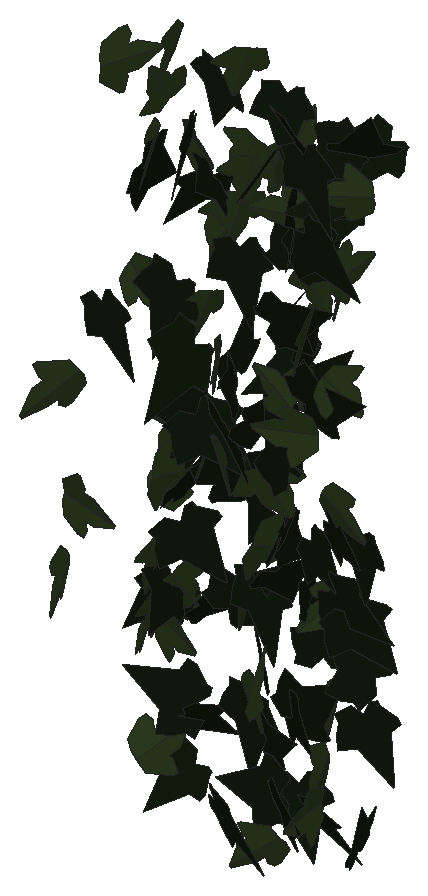
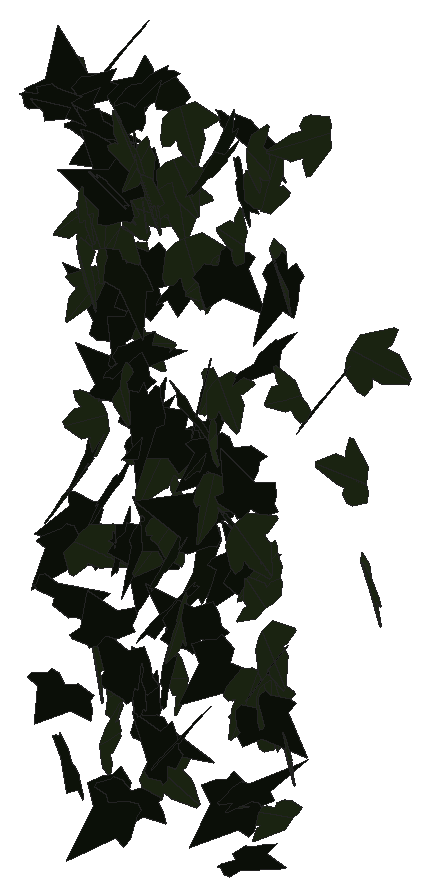
# SketchUp Ruby script. Lengths in inches.
U = 1.inch
M = Sketchup.active_model
def pt(a) = Geom::Point3d.new(a.map { |v| v * U })
def face(e, loops, mat)
  f = e.add_face(loops[0].map { |a| pt(a) })
  loops[1..].each { |l| e.add_face(l.map { |a| pt(a) }).erase! }
  f.material = f.back_material = mat if mat
  f
end
# faces: each face lists its corners as indices into pts; further lists are holes
def faces(e, pts, list, mat = nil) = list.each { |f| face(e, (f[0].is_a?(Array) ? f : [f]).map { |l| l.map { |i| pts[i] } }, mat) }
# xy, xz, yz: faces in a plane at the given z, y or x. An outline is a flat list of corners, or four numbers for a rectangle; further outlines are holes
def ring(l) = l.size == 4 ? [[l[0], l[1]], [l[2], l[1]], [l[2], l[3]], [l[0], l[3]]] : l.each_slice(2).to_a
def flat(e, list, mat, &to3) = list.each { |f| face(e, (f[0].is_a?(Array) ? f : [f]).map { |l| ring(l).map { |u, v| to3.(u, v) } }, mat) }
def xy(e, z, list, mat = nil) = flat(e, list, mat) { |x, y| [x, y, z] }
def xz(e, y, list, mat = nil) = flat(e, list, mat) { |x, z| [x, y, z] }
def yz(e, x, list, mat = nil) = flat(e, list, mat) { |y, z| [x, y, z] }
def lines(e, pts, list) = list.each { |a, b| e.add_line(pt(pts[a]), pt(pts[b])) }
# prism: a flat outline (further loops are holes) pulled along v
def prism(e, loops, v, mat = nil)
  f = face(e, loops, mat); d = Geom::Vector3d.new(v.map { |x| x * U })
  f.pushpull(f.normal.samedirection?(d) ? d.length : -d.length)
end
def box(e, o, s, mat = nil) = prism(e, [[o, [o[0] + s[0], o[1], o[2]], [o[0] + s[0], o[1] + s[1], o[2]], [o[0], o[1] + s[1], o[2]]]], [0, 0, s[2]], mat)
def at(x, y, z, deg = 0) = Geom::Transformation.translation(pt([x, y, z])) * Geom::Transformation.rotation(ORIGIN, Z_AXIS, deg.degrees)
def axes(o, x, y, z) = Geom::Transformation.new([*x, 0, *y, 0, *z, 0, *pt(o).to_a, 1])
def part(name) = M.definitions.add(name)
# library, detail: a bought-in or finely detailed component or shape, given as its bounding box
def library(name, o, s) = part(name).tap { |d| box(d.entities, o, s) }
def detail(e, o, s) = box(e.add_group.entities, o, s)
def put(e, d, t, mat = nil) = e.add_instance(d, t).tap { |i| i.material = mat if mat }
def group(e, t, mat = nil) = e.add_group.tap { |g| g.transformation = t; g.material = mat if mat }.entities
root = M.entities
M.materials.add("efeu1").color = [18, 25, 13]
M.materials.add("efeu2").color = [43, 57, 29]
c1 = part("ivyleaf_9")
p = [[1.54,2.16,1.25],[1.36,2.04,1.19],[-0.21,0.99,0.68],[-0.71,1.11,0.82],[-0.85,0.86,0.67],[-0.8,0.17,0.21],
  [-0.9,-0.01,0.1],[-0.67,-0.16,-0.02],[-0.08,-0.08,-0.05],[-0.03,-0.6,-0.4],[0.65,-0.88,-0.66],[0.83,-0.6,-0.49],
  [1.29,-0.42,-0.43],[1.8125,-0.07,-0.26],[1.21,0.44,0.15]]
faces(c1.entities,p,[[0,1,2,3,4,5,6,7,8,9,10,11,12,13,14]],"efeu1")
c2 = part("ivyleaf_10")
p = [[0,0.5,-0.03],[-0.0625,2.02,-0.43],[-0.19,2.01,-0.46],[-0.54,1.05,-0.29],[-0.52,0.625,-0.18],[-0.83,0.76,-0.28],
  [-1.16,0.64,-0.33],[-1.15,0.33,-0.24],[-0.77,-0.39,0.02],[-0.3,-0.51,0.16],[0.04,-0.48,0.23],[-0.02,2.01,-0.4375],
  [-0.06,2.01,-0.43],[0.04,-0.49,0.23],[0.67,-0.49,0.14],[1.38,0.36,-0.2],[1.375,0.51,-0.24],[0.81,0.65,-0.19],
  [0.62,0.59,-0.15],[0.6,1.09,-0.28],[0.5,1.23,-0.31]]
faces(c2.entities,p,[[0,1,2,3,4,5,6,7,8,9,10],[11,12,0,13,14,15,16,17,18,19,20]],"efeu2")
put(root,c1,axes([575.81,114.26,235.49],[-1.308,-0.18364,-0.30773],[0.30435,0.04552,-1.32082],[0.18917,-1.34294,-0.00269]))
put(root,c1,axes([577.29,114.21,213.41],[1.13881,-0.56952,-0.46488],[-0.40509,0.22917,-1.27308],[0.61349,1.2085,0.02233]))
put(root,c2,axes([577.51,116.32,217.81],[0.87571,-0.89625,-0.03596],[0.02653,-0.02436,1.25304],[-0.89657,-0.87611,0.00195]))
put(root,c2,axes([566.08,117.8,228.98],[-0.23963,-0.68527,1.0215],[-0.33171,-0.96615,-0.72595],[1.1845,-0.4092,0.00335]))
put(root,c2,axes([566.27,117.97,222.96],[0.05434,-0.11388,1.24145],[1.24187,0.11376,-0.04392],[-0.10916,1.23742,0.11829]))
put(root,c2,axes([565.16,118.66,218.99],[0.88338,-0.86872,0.00346],[0.01078,0.00603,-1.23891],[0.86866,0.88336,0.01186]))
put(root,c2,axes([578.02,119.21,229.83],[0.07725,-0.00335,-1.1407],[-1.13047,-0.15301,-0.0761],[-0.15244,1.13303,-0.01366]))
put(root,c2,axes([577.11,121.18,210.1],[-0.02306,0.08063,-1.16362],[-0.17029,-1.15161,-0.07642],[-1.15391,0.16833,0.03453]))
put(root,c1,axes([575.34,121.03,209.32],[0.20393,-0.35155,1.12904],[0.49116,-1.01702,-0.40539],[1.07568,0.53102,-0.02895]))
put(root,c2,axes([572.17,120.58,226.52],[-0.60926,0.6898,-0.52411],[0.35827,-0.38277,-0.92024],[-0.78877,-0.70666,-0.01315]))
put(root,c1,axes([576.48,121.25,242],[0.52528,-1.1541,-0.11164],[-0.03269,0.10778,-1.26793],[1.15902,0.52608,0.01483]))
put(root,c1,axes([574.41,120.85,240.82],[-0.57801,0.89862,-0.10934],[0.06117,-0.09065,-1.06846],[-0.90318,-0.58123,-0.00239]))
put(root,c2,axes([574.33,121.5,207.34],[-0.49806,-0.4723,0.85777],[-0.6544,-0.55534,-0.68575],[0.72842,-0.82184,-0.02956]))
put(root,c1,axes([570.8,121.91,238.82],[0.68254,-0.51553,-0.61479],[0.47628,-0.38921,0.85514],[-0.64567,-0.83207,-0.01909]))
put(root,c1,axes([576.15,121.74,237.82],[-0.09742,-0.10391,-1.25306],[1.06381,0.66316,-0.1377],[0.67026,-1.06764,0.03642]))
put(root,c1,axes([575.94,122.14,229.29],[0.24138,-0.11874,1.26812],[1.03688,-0.73122,-0.26583],[0.73965,1.06381,-0.04118]))
put(root,c1,axes([574.28,122.06,209.54],[-0.49487,-0.25561,-1.00449],[-0.90234,-0.44148,0.55688],[-0.51003,1.02908,-0.0106]))
put(root,c2,axes([575.52,122.59,233.08],[0.64784,-1.01004,0.30154],[0.16038,-0.25537,-1.19995],[1.04181,0.6674,-0.00279]))
put(root,c2,axes([578.47,122.65,240.23],[-0.09478,-0.03356,1.07827],[-0.8651,-0.64432,-0.09609],[0.64452,-0.86977,0.02958]))
put(root,c1,axes([575.39,122.17,235.97],[-0.41369,-0.0999,1.16594],[1.15981,-0.19954,0.39442],[0.15569,1.22096,0.15985]))
put(root,c1,axes([564.27,122.58,229.89],[0.58046,-1.04021,-0.20961],[-0.08507,0.19253,-1.19105],[1.0577,0.58634,0.01924]))
put(root,c2,axes([571.95,123.02,213.44],[-0.38856,0.41482,-0.98164],[0.64624,-0.73911,-0.56813],[-0.84739,-0.75387,0.01685]))
put(root,c2,axes([576.77,122.79,224.47],[-0.59437,0.29702,-0.96008],[0.88022,-0.38438,-0.66385],[-0.48494,-1.06173,-0.02824]))
put(root,c2,axes([577.25,122.11,230.68],[0.27661,0.76003,0.69866],[0.16133,0.68259,-0.80643],[-1.01968,0.31417,0.06194]))
put(root,c2,axes([574.28,122.6,228.75],[0.51065,0.17477,0.90056],[-0.90498,-0.07277,0.52728],[0.15019,-1.0327,0.11525]))
put(root,c1,axes([570.17,123.55,225.62],[0.51802,-0.87592,0.7521],[0.35289,-0.66475,-1.01725],[1.09925,0.62617,-0.02786]))
put(root,c1,axes([576.83,122.6,223.37],[0.78768,-0.39827,-0.60365],[-0.49643,0.35129,-0.87955],[0.5259,0.92813,0.07387]))
put(root,c1,axes([574.97,122.33,238.24],[-0.05459,-0.00295,-1.46886],[-1.41813,0.38306,0.05193],[0.38269,1.41908,-0.01708]))
put(root,c1,axes([573.45,122.9,232.125],[1.02167,0.21551,-0.642],[0.51591,0.50504,0.99055],[0.43868,-1.09586,0.33025]))
put(root,c1,axes([577.37,123.37,239.05],[-0.82595,0.02987,0.6706],[-0.67115,-0.01689,-0.82588],[-0.01253,-1.06378,0.03195]))
put(root,c1,axes([575.58,122.92,221.87],[0.57534,-0.68369,-0.57412],[-0.35559,0.451,-0.89342],[0.8189,0.67618,0.01541]))
put(root,c1,axes([568.46,122.78,220.45],[0.02167,-0.63779,-0.98844],[0.02664,0.98862,-0.63733],[1.17605,-0.01064,0.03265]))
put(root,c1,axes([573.6,123.6,241.25],[0.61528,-0.59217,0.85144],[0.59313,-0.61121,-0.8537],[0.85078,0.85437,-0.02059]))
put(root,c2,axes([564.87,122.43,242.25],[0.03814,-0.06329,-1.22483],[0.68128,1.02007,-0.03149],[1.01984,-0.67907,0.06685]))
put(root,c1,axes([573.7,123.65,212.94],[0.15404,-0.15283,-1.02701],[1.03826,0.01201,0.15395],[-0.01067,-1.03843,0.15293]))
put(root,c2,axes([572.9,123.05,224.27],[-0.96525,-0.68544,-0.45912],[0.3658,0.2778,-1.18378],[0.73947,-1.03215,-0.01371]))
put(root,c1,axes([568.125,123.8,239.58],[-0.59459,0.14311,-0.93716],[0.86245,-0.37766,-0.60485],[-0.39363,-1.04364,0.09037]))
put(root,c1,axes([566.93,124.16,231.18],[-0.16984,-1.18488,0.38736],[-0.08949,-0.37834,-1.19653],[1.24338,-0.18908,-0.03321]))
put(root,c1,axes([573.8,123.35,224.81],[-0.25865,-1.05824,0.68082],[0.22994,0.6436,1.08774],[-1.23714,0.34087,0.05983]))
put(root,c1,axes([570.34,124.05,227.08],[-0.13417,0.03617,1.01376],[-0.06455,-1.02082,0.02788],[1.01235,-0.06029,0.13614]))
put(root,c1,axes([576.36,123.26,219.56],[0.1442,-0.06873,-1.20958],[0.98645,0.71386,0.07704],[0.70338,-0.98706,0.13994]))
put(root,c1,axes([569.0625,123.21,225.74],[0.0059,-0.60676,-1.09595],[0.46315,1.01936,-0.56186],[1.16394,-0.40255,0.22913]))
put(root,c1,axes([575.25,122.99,218.52],[-0.04556,-0.39737,0.98233],[0.15245,0.97055,0.39967],[-1.04863,0.15836,0.01543]))
put(root,c1,axes([576.49,124.28,241.17],[-0.59224,-0.62701,0.63319],[-0.44583,-0.4498,-0.8624],[0.77157,-0.74119,-0.01229]))
put(root,c1,axes([574.2,123.5625,212.57],[-0.26894,0.16016,1.1879],[0.97584,-0.67772,0.3123],[0.69606,1.012,0.02114]))
put(root,c1,axes([573.18,124.07,242.68],[-0.13412,-1.04425,-0.11183],[0.01371,0.11099,-1.05282],[1.05013,-0.13482,-0.00053]))
put(root,c2,axes([566.43,122.92,208.47],[0.62396,0.16446,-0.9582],[0.61581,0.81418,0.54075],[0.75231,-0.80286,0.3521]))
put(root,c2,axes([576.24,124.18,218.99],[0.55697,0.4708,-0.95349],[-0.71553,-0.63032,-0.72919],[-0.78665,0.90667,-0.01183]))
put(root,c1,axes([573.4375,123.19,219.62],[0.47403,0.92692,-0.14562],[-0.08794,-0.11854,-1.04082],[-0.93416,0.48152,0.02409]))
put(root,c1,axes([566.35,124.57,215.85],[-0.05988,-0.83575,0.70239],[-0.05038,-0.70059,-0.83789],[1.09055,-0.07825,-0.00014]))
put(root,c2,axes([574.76,124.58,209.89],[0.03578,-0.37054,1.19304],[0.7321,-0.96089,-0.32039],[1.01226,0.70804,0.18955]))
put(root,c1,axes([577.23,123.54,218.66],[-0.03623,-0.58858,-0.97281],[0.17497,0.95882,-0.58664],[1.12346,-0.16831,0.05999]))
put(root,c1,axes([570.58,124.16,234.08],[0.07411,-1.12983,-0.26375],[-0.03342,0.2621,-1.13215],[1.15972,0.07976,-0.01577]))
put(root,c2,axes([574.89,123.86,234.38],[-1.04672,-0.12524,-0.14372],[0.1435,0.01044,-1.05417],[0.1255,-1.05649,0.00662]))
put(root,c2,axes([572.39,123.25,220.67],[-0.21299,-0.66723,-1.05474],[0.32058,1.00485,-0.7004],[1.2062,-0.38488,-0.0001]))
put(root,c1,axes([570.74,124.75,211.52],[0.11836,-1.17167,0.39629],[0.08579,-0.38937,-1.17682],[1.2339,0.13947,0.04381]))
put(root,c2,axes([575.92,123.92,213.875],[0.64741,-0.81978,-0.44762],[-0.201,0.40959,-1.04085],[0.91214,0.67211,0.08834]))
put(root,c2,axes([565.97,124.47,217.86],[0.12122,-1.13641,0.33175],[0.06889,-0.32615,-1.14239],[1.18184,0.13558,0.03256]))
put(root,c1,axes([577.93,124.05,215.74],[-1.08954,-0.36109,-0.56654],[-0.53339,-0.19137,1.14775],[-0.40848,1.21303,0.01243]))
put(root,c1,axes([577.73,123.37,207.38],[-0.06505,0.55061,0.92319],[-0.19467,0.90356,-0.55261],[-1.05715,-0.20027,0.04495]))
put(root,c1,axes([573.6,125.05,229.25],[-0.57059,-0.59166,0.84111],[-0.56536,-0.62302,-0.82178],[0.85901,-0.80305,0.01784]))
put(root,c1,axes([570.24,123.95,216.5],[-0.312,0.09261,1.06489],[1.04259,-0.21825,0.32444],[0.2357,1.08798,-0.02556]))
put(root,c1,axes([571.32,124.66,217.72],[0.26866,-1.24201,-0.01926],[-0.00403,0.01883,-1.27073],[1.24215,0.26869,0.00004]))
put(root,c1,axes([573.16,123.42,220.6875],[0.04988,0.51626,0.91873],[-0.14559,0.91432,-0.50587],[-1.04374,-0.10287,0.11447]))
put(root,c2,axes([565.99,124.82,239.99],[-0.2649,-0.86215,-0.63928],[-0.19612,-0.60849,0.9019],[-1.05524,0.32952,-0.00715]))
put(root,c1,axes([571.51,124.61,210.07],[0.13303,-0.1585,1.03006],[0.67895,-0.77464,-0.20688],[0.79068,0.69185,0.00434]))
put(root,c1,axes([576.64,124.93,221.66],[0.24267,-1.05378,0.43407],[0.09227,-0.42418,-1.08135],[1.13594,0.25957,-0.0049]))
put(root,c2,axes([573.39,124.53,236.67],[-0.00409,0.02885,1.12319],[-1.02444,-0.46136,0.00812],[0.46142,-1.02407,0.02798]))
put(root,c1,axes([572.1,124.01,213.4375],[0.06219,-0.48274,0.92118],[-0.16482,0.90659,0.48622],[-1.02686,-0.17475,-0.02225]))
put(root,c1,axes([567.2,125.05,207.0625],[-0.63475,-0.67927,0.40065],[-0.24748,-0.31675,-0.92912],[0.74879,-0.68051,0.03256]))
put(root,c1,axes([574.18,123.88,233.26],[-0.35907,1.08501,0.13916],[-0.04935,0.13024,-1.14286],[-1.09278,-0.36239,0.00589]))
put(root,c1,axes([576.75,124.54,240.81],[0.97116,0.44547,0.31863],[-0.2871,-0.13833,1.06844],[0.46642,-1.01269,-0.00578]))
put(root,c2,axes([565.98,124.61,213.86],[0.0748,-0.098,1.21389],[1.21074,-0.12512,-0.08471],[0.13129,1.20974,0.08957]))
put(root,c2,axes([570.99,124.52,239.3],[-0.83868,-0.19977,0.58892],[-0.5421,-0.24965,-0.85669],[0.30473,-0.99393,0.09681]))
put(root,c1,axes([566.89,124.3,220.66],[0.26371,0.92298,0.30225],[-0.09728,-0.28652,0.95981],[0.96632,-0.28072,0.01414]))
put(root,c2,axes([570.875,124.6,238.27],[-0.68653,-0.76689,0.17145],[-0.10252,-0.13831,-1.02918],[0.77911,-0.69397,0.01565]))
put(root,c2,axes([569.34,124.11,224.15],[-0.0626,-0.98771,-0.66786],[0.07012,0.66457,-0.98942],[1.19024,-0.09109,0.02316]))
put(root,c2,axes([565.8,124.6875,215.33],[0.13493,-1.17504,0.03833],[0.0032,-0.03822,-1.18276],[1.17566,0.13496,-0.00118]))
put(root,c1,axes([571.33,123.7,226.15],[-0.03283,0.38685,-0.9635],[-0.07516,0.96056,0.38823],[1.03554,0.08199,-0.00237]))
put(root,c2,axes([564.39,124.62,230.62],[0.55501,0.08963,0.93672],[0.93279,0.09088,-0.56138],[-0.12398,1.085,-0.03036]))
put(root,c1,axes([569.47,123.91,222.37],[0.2032,0.0841,1.23687],[1.14298,0.47271,-0.21991],[-0.48013,1.1609,-0.00006]))
put(root,c1,axes([567.08,125.25,210.06],[-0.36472,-1.1102,-0.37263],[-0.11558,-0.35426,1.16857],[-1.16535,0.3826,0.00073]))
put(root,c2,axes([576.48,123.79,235.15],[0.0692,-0.06917,-1.13677],[0.21092,1.11995,-0.05531],[1.11917,-0.20679,0.08071]))
put(root,c2,axes([564.95,124.67,213.61],[0.59936,-0.76134,-0.25243],[-0.15469,0.19949,-0.96896],[0.78704,0.619,0.00179]))
put(root,c2,axes([569.39,123.84,234.4375],[0.12136,0.0758,-1.11438],[0.12485,1.11299,0.0893],[1.10996,-0.13348,0.1118]))
put(root,c1,axes([573.21,124.89,208.19],[-0.56053,-0.56211,-0.83031],[0.65344,0.51672,-0.79094],[0.76052,-0.85826,0.06761]))
put(root,c1,axes([566.84,124.69,224.41],[-0.58287,-0.03055,0.83181],[0.81041,-0.25252,0.5586],[0.18991,0.98381,0.16921]))
put(root,c2,axes([569.9,125.04,235.91],[-0.58782,-1.08665,0.27018],[-0.12667,-0.23865,-1.23545],[1.11254,-0.60131,0.00209]))
put(root,c1,axes([572.99,124.26,220.79],[0.20457,-0.17743,-1.01776],[-0.77834,0.65577,-0.27077],[0.67934,0.80477,-0.00375]))
put(root,c2,axes([570.88,124.1,217.43],[0.20242,-0.55887,-1.09726],[-0.09395,1.10174,-0.57848],[1.2278,0.17644,0.13664]))
put(root,c2,axes([566.18,124.03,221.5625],[0.01457,-0.40498,-1.16165],[0.20795,1.14583,-0.39685],[1.21252,-0.19165,0.08202]))
put(root,c2,axes([574.39,124.65,228.375],[-0.83542,0.14601,0.82284],[-0.81664,0.10438,-0.84765],[-0.17742,-1.16794,0.02711]))
put(root,c2,axes([564.95,125.16,237.3],[0.74317,-1.01173,0.08716],[0.05111,-0.07061,-1.25534],[1.01419,0.74492,-0.00061]))
put(root,c1,axes([568.46,124.15,215.82],[0.51062,0.67719,0.56864],[0.31005,0.47784,-0.84747],[-0.82813,0.59645,0.03333]))
put(root,c1,axes([573.69,124.63,227.81],[-0.31721,-0.00406,1.00677],[1.00664,0.01593,0.31724],[-0.01641,1.05544,-0.00091]))
put(root,c2,axes([568.18,125.56,227.54],[0.24849,-0.25048,0.96234],[0.70256,-0.65777,-0.35262],[0.70374,0.74511,0.01222]))
put(root,c2,axes([565.83,125.62,242.39],[0.37293,-0.78141,0.76922],[0.36468,-0.67784,-0.86539],[1.03407,0.52086,0.02779]))
put(root,c1,axes([574.75,124.71,215.375],[-0.65046,-0.35059,0.76086],[0.67188,0.35705,0.73892],[-0.50039,0.93516,0.00312]))
put(root,c1,axes([570.47,125.97,220.55],[-0.10285,-0.69461,0.89319],[0.11156,-0.89873,-0.68607],[1.12598,0.0256,0.14956]))
put(root,c1,axes([577.58,125.6,241.26],[-0.88696,-0.494,0.0921],[-0.08353,-0.03928,-1.01523],[0.49552,-0.89086,-0.0063]))
put(root,c1,axes([573.83,124.53,229.97],[-0.08523,-0.32975,1.00135],[0.34344,0.94113,0.33915],[-0.99673,0.35248,0.03124]))
put(root,c1,axes([574.44,125.36,237.92],[-1.01631,0.07176,-0.20999],[0.21034,-0.00236,-1.01876],[-0.07075,-1.03777,-0.01221]))
put(root,c1,axes([572.5,124.68,227.66],[0.8475,0.1121,-0.95635],[-0.95933,-0.01119,-0.85146],[-0.08275,1.27779,0.07644]))
put(root,c1,axes([567.67,125.03,223.55],[-0.83165,0.55974,0.19008],[-0.1587,0.10464,-1.00247],[-0.56943,-0.84666,0.00177]))
put(root,c2,axes([572.75,124.42,239.47],[0.02494,-0.41064,-0.96815],[0.0642,0.96721,-0.40859],[1.04967,-0.0494,0.04799]))
put(root,c1,axes([573.7,124.78,207.47],[1.28038,-0.07869,-0.0774],[-0.07726,0.0047,-1.2828],[0.07883,1.28271,-0.00004]))
put(root,c1,axes([573.33,125,237.38],[0.44525,-0.1165,1.03505],[1.01098,-0.22256,-0.45994],[0.25066,1.10456,0.01649]))
put(root,c2,axes([574.36,125.07,237.06],[-1.01432,-0.36403,0.04194],[-0.03949,-0.01411,-1.07767],[0.3643,-1.01509,-0.00006]))
put(root,c1,axes([567.79,125.49,236.15],[-0.14693,0.51781,-0.87248],[-0.01982,-0.88288,-0.52065],[-1.01438,-0.05775,0.13655]))
put(root,c2,axes([567.7,125.43,230.12],[-0.24641,-0.95582,0.27345],[-0.0694,-0.2645,-0.98707],[0.99174,-0.256,-0.00113]))
put(root,c2,axes([566.75,125.45,237.74],[0.04451,-0.20955,0.99847],[0.99916,-0.19306,-0.08506],[0.20621,0.98064,0.19662]))
put(root,c1,axes([565.625,125.57,215.2],[0.11388,0.29858,-0.99083],[-0.3325,-0.93341,-0.31949],[-0.97997,0.35139,-0.00674]))
put(root,c2,axes([572.81,125.26,239.52],[1.01493,-0.42771,-0.4023],[0.37096,-0.15568,1.10137],[-0.45517,-1.0806,0.00056]))
put(root,c1,axes([565.06,124.4375,236.36],[-0.00799,-0.03304,-1.24456],[-0.83149,0.92646,-0.01926],[0.92662,0.83106,-0.02801]))
put(root,c2,axes([575.1875,125.34,237],[0.15477,-1.02543,-0.10195],[-0.01617,0.10066,-1.03704],[1.03036,0.15561,-0.00097]))
put(root,c2,axes([572.02,125.23,238.55],[0.79795,-0.52664,-0.39578],[-0.28232,0.28831,-0.95283],[0.59522,0.84276,0.07864]))
put(root,c1,axes([567.28,124.69,209.74],[0.79292,0.55786,0.29525],[0.232,0.18329,-0.96937],[-0.58699,0.82601,0.0157]))
put(root,c1,axes([569.99,124.66,227.95],[-0.88427,0.61344,-0.33012],[-0.2797,0.17594,1.07612],[0.63801,0.92734,0.01421]))
put(root,c1,axes([567.91,126.19,240.86],[-0.05265,-0.90569,0.67551],[0.23761,-0.67,-0.87977],[1.10459,0.10095,0.22144]))
put(root,c1,axes([576.43,125.43,212.5],[-0.37792,-0.46471,-0.9378],[0.69727,0.63178,-0.59406],[0.78053,-0.78939,0.07662]))
put(root,c2,axes([569.75,125.6,242.81],[-0.55809,-0.86661,0.25518],[-0.14536,-0.20989,-1.03073],[0.89162,-0.57665,-0.00831]))
put(root,c2,axes([565.9,124.9,220.08],[0.32642,0.76329,-0.56949],[0.22258,0.52419,0.83016],[0.92596,-0.39509,0.00121]))
put(root,c2,axes([575.2,125.67,234.04],[0.63875,-1.02807,0.04551],[0.02074,-0.04069,-1.21034],[1.02887,0.63908,-0.00386]))
put(root,c2,axes([566.31,125.0625,215.97],[-0.46015,-0.9413,-0.64512],[0.24608,0.59738,-1.04716],[1.1143,-0.52063,-0.03515]))
put(root,c2,axes([566.09,126.03,223.78],[-0.13871,-1.04651,0.60457],[-0.07411,-0.60003,-1.05565],[1.20631,-0.1572,0.00466]))
